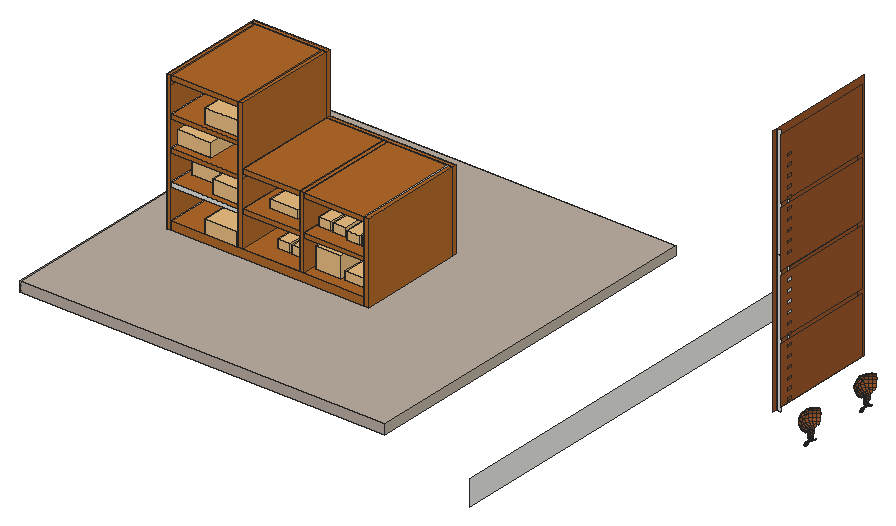
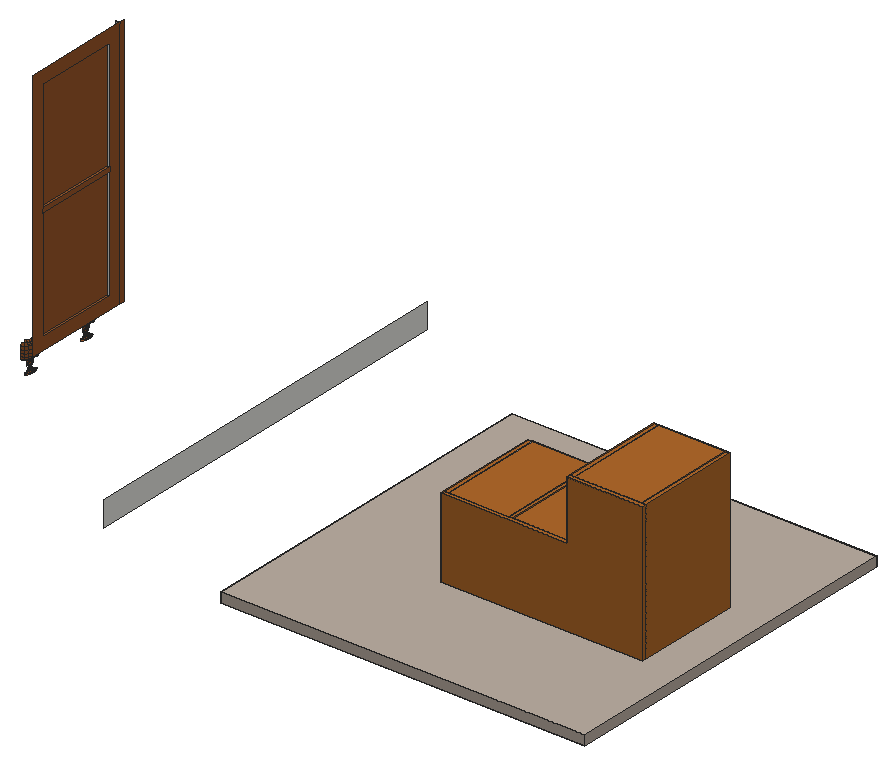
# SketchUp Ruby script. Lengths in inches.
U = 1.inch
M = Sketchup.active_model
def pt(a) = Geom::Point3d.new(a.map { |v| v * U })
def face(e, loops, mat)
  f = e.add_face(loops[0].map { |a| pt(a) })
  loops[1..].each { |l| e.add_face(l.map { |a| pt(a) }).erase! }
  f.material = f.back_material = mat if mat
  f
end
# faces: each face lists its corners as indices into pts; further lists are holes
def faces(e, pts, list, mat = nil) = list.each { |f| face(e, (f[0].is_a?(Array) ? f : [f]).map { |l| l.map { |i| pts[i] } }, mat) }
# xy, xz, yz: faces in a plane at the given z, y or x. An outline is a flat list of corners, or four numbers for a rectangle; further outlines are holes
def ring(l) = l.size == 4 ? [[l[0], l[1]], [l[2], l[1]], [l[2], l[3]], [l[0], l[3]]] : l.each_slice(2).to_a
def flat(e, list, mat, &to3) = list.each { |f| face(e, (f[0].is_a?(Array) ? f : [f]).map { |l| ring(l).map { |u, v| to3.(u, v) } }, mat) }
def xy(e, z, list, mat = nil) = flat(e, list, mat) { |x, y| [x, y, z] }
def xz(e, y, list, mat = nil) = flat(e, list, mat) { |x, z| [x, y, z] }
def yz(e, x, list, mat = nil) = flat(e, list, mat) { |y, z| [x, y, z] }
def lines(e, pts, list) = list.each { |a, b| e.add_line(pt(pts[a]), pt(pts[b])) }
# prism: a flat outline (further loops are holes) pulled along v
def prism(e, loops, v, mat = nil)
  f = face(e, loops, mat); d = Geom::Vector3d.new(v.map { |x| x * U })
  f.pushpull(f.normal.samedirection?(d) ? d.length : -d.length)
end
def box(e, o, s, mat = nil) = prism(e, [[o, [o[0] + s[0], o[1], o[2]], [o[0] + s[0], o[1] + s[1], o[2]], [o[0], o[1] + s[1], o[2]]]], [0, 0, s[2]], mat)
def at(x, y, z, deg = 0) = Geom::Transformation.translation(pt([x, y, z])) * Geom::Transformation.rotation(ORIGIN, Z_AXIS, deg.degrees)
def axes(o, x, y, z) = Geom::Transformation.new([*x, 0, *y, 0, *z, 0, *pt(o).to_a, 1])
def part(name) = M.definitions.add(name)
# library, detail: a bought-in or finely detailed component or shape, given as its bounding box
def library(name, o, s) = part(name).tap { |d| box(d.entities, o, s) }
def detail(e, o, s) = box(e.add_group.entities, o, s)
def put(e, d, t, mat = nil) = e.add_instance(d, t).tap { |i| i.material = mat if mat }
def group(e, t, mat = nil) = e.add_group.tap { |g| g.transformation = t; g.material = mat if mat }.entities
root = M.entities
M.materials.add("[Color A01]").color = [255, 204, 204]
M.materials.add("[Color A07]").color = [153, 0, 0]
M.materials.add("[Color E01]").color = [255, 255, 204]
M.materials.add("[Color G05]").color = [0, 255, 0]
M.materials.add("[Color I01]").color = [204, 204, 255]
M.materials.add("[Color J06]").color = [102, 0, 204]
M.materials.add("[Color K04]").color = [255, 50, 255]
M.materials.add("[Color L11]").color = [153, 0, 76]
M.materials.add("[Color L16]").color = [102, 0, 51]
M.materials.add("[Color M01]").color = [226, 226, 226]
M.materials.add("[Encaustic Tile Circular 02]").color = [187, 174, 162]
M.materials.add("[Wood Bamboo]").color = [177, 105, 43]
M.materials.add("[Wood Cherry Original]").color = [152, 86, 42]
c1 = library("Group\#29",[0,0,0],[10.56,11.41,4.2])
c2 = library("12.1shooters 6",[-12.32,-1,-0.41],[13.09,17.1,6.95])
c3 = library("Group\#37",[0,0,0],[11.84,13.47,5.24])
c4 = library("Group\#20",[0,0,0],[10.15,12.29,4.29])
c5 = library("Group\#27",[0,0,0],[11.1875,13.6,5.13])
c6 = library("Group\#4",[0,0,0],[9.05,3.05,1.93])
c7 = library("Group\#47",[0,0,0],[9.05,6.59,1.93])
c8 = library("Group\#2",[0,0,0],[9.05,3.05,1.93])
c9 = library("Group\#75",[0,0,0],[9.05,3.05,1.93])
c10 = library("ZSHOE",[-0.73,-0.58,0],[16.86,13.33,10.8125])
c11 = library("Group\#12",[0,0,0],[9.05,3.05,1.93])
c12 = library("Group\#3",[0,0,0],[9.05,3.05,1.93])
c13 = library("Group\#44",[0,0,0],[9.05,6.59,1.93])
c14 = library("Group\#73",[0,0,0],[9.05,3.05,1.93])
xy(root,0,[[8.92,47.18,9.92,72.18],[9.92,47.18,9.92,72.18,8.92,72.18,8.92,73.18,56.92,73.18,56.92,72.18,55.92,72.18,55.92,47.18],[55.92,47.18,56.92,72.18]])
xy(root,2,[[25.92,47.18,26.92,72.18],[40.48,47.18,41.48,72.18]])
xy(root,2,[[9.92,47.18,25.92,72.18],[26.92,47.18,40.48,72.18],[41.48,47.18,55.92,72.18]],"[Wood Bamboo]")
xy(root,6,[[159.72,48.4,159.8125,48.51,159.45,48.88,159.33,48.79],[159.33,48.79,159.45,48.88,159.1875,49.33,159.05,49.28],[159.05,49.28,159.1875,49.33,159.06,49.84,158.91,49.82],[158.91,49.82,159.06,49.84,159.06,50.35,158.91,50.375],[159.06,50.35,159.19,50.85,159.06,50.91,158.91,50.375],
  [159.19,50.85,159.46,51.3,159.34,51.4,159.06,50.91],[159.46,51.3,159.82,51.67,159.73,51.79,159.34,51.4],[159.72,65.02,159.8125,65.14,159.45,65.51,159.33,65.42],[159.33,65.42,159.45,65.51,159.1875,65.96,159.05,65.9],[159.05,65.9,159.1875,65.96,159.06,66.46,158.91,66.44],
  [158.91,66.44,159.06,66.46,159.06,66.98,158.91,67],[159.06,66.98,159.19,67.48,159.06,67.54,158.91,67],[159.19,67.48,159.46,67.93,159.34,68.02,159.06,67.54],[159.46,67.93,159.82,68.29,159.73,68.41,159.34,68.02]],"[Wood Cherry Original]")
xy(root,9.25,[[9.92,47.18,25.92,72.18]])
xy(root,9.5,[[41.48,47.18,55.92,72.18]])
xy(root,9.5,[[26.92,47.18,40.48,72.18]],"[Wood Bamboo]")
xy(root,10.25,[[9.92,47.18,25.92,72.18]],"[Wood Bamboo]")
xy(root,10.5,[[26.92,47.18,40.48,72.18],[41.48,47.18,55.92,72.18]],"[Wood Bamboo]")
xy(root,16.08,[[154.9,49.11,155.65,69.11]],"[Wood Cherry Original]")
xy(root,16.5,[[9.92,47.18,25.92,72.18]],"[Wood Bamboo]")
xy(root,17.5,[[9.92,47.18,25.92,72.18]],"[Wood Bamboo]")
xy(root,19,[[26.92,47.18,40.48,72.18],[40.48,47.18,41.48,72.18],[41.48,47.18,55.92,72.18],[55.92,47.18,56.92,72.18],[26.92,72.18,56.92,73.18]],"[Wood Bamboo]")
xy(root,23.75,[[9.92,47.18,25.92,72.18]],"[Wood Bamboo]")
xy(root,24.75,[[9.92,47.18,25.92,72.18]],"[Wood Bamboo]")
xy(root,33,[[8.92,47.18,9.92,72.18],[9.92,47.18,25.92,72.18],[25.92,47.18,26.92,72.18],[8.92,72.18,25.92,73.18],[25.92,72.18,26.92,73.18]],"[Wood Bamboo]")
xy(root,42.58,[[154.9,49.11,155.65,69.11]],"[Wood Cherry Original]")
xy(root,43.58,[[154.9,49.11,155.65,69.11]],"[Wood Cherry Original]")
xy(root,70.08,[[154.9,49.11,155.65,69.11]])
xz(root,46.11,[[154.9,13.08,155.9,46.26],[154.9,46.26,155.9,73.08]])
xz(root,47.18,[[9.92,9.25,25.92,10.25]])
xz(root,47.18,[[8.92,0,9.92,33],[9.92,0,55.92,2],[55.92,0,56.92,19],[25.92,2,26.92,33],[40.48,2,41.48,19],
  [26.92,9.5,40.48,10.5],[41.48,9.5,55.92,10.5],[9.92,16.5,25.92,17.5],[26.92,18,40.48,19],[41.48,18,55.92,19],
  [9.92,23.75,25.92,24.75],[9.92,32,25.92,33]],"[Wood Bamboo]")
xz(root,49.11,[[154.9,16.08,155.65,42.58],[154.9,43.58,155.65,70.08]])
xz(root,69.11,[[154.9,16.08,155.65,42.58],[154.9,43.58,155.65,70.08]],"[Wood Cherry Original]")
xz(root,72.18,[[8.92,0,9.92,33],[55.92,0,56.92,19],[25.92,2,26.92,33],[40.48,2,41.48,2,41.48,17,26.92,17,26.92,9.5,40.48,9.5],[9.92,9.25,25.92,31],
  [41.48,9.5,55.92,17],[26.92,17,40.48,19],[40.48,17,41.48,19],[41.48,17,55.92,19],[9.92,17.5,25.92,23.75],
  [9.92,31,25.92,33]])
xz(root,72.18,[[9.92,2,25.92,9.25],[26.92,2,40.48,9.5],[41.48,2,55.92,9.5],[9.92,10.25,25.92,16.5],[26.92,10.5,40.48,17],
  [41.48,10.5,55.92,17],[9.92,24.75,25.92,31]],"[Wood Bamboo]")
xz(root,73.18,[[8.92,0,8.92,33,26.92,33,26.92,19,56.92,19,56.92,0]],"[Wood Bamboo]")
yz(root,8.92,[[47.18,0,72.18,33],[72.18,0,73.18,33]],"[Wood Bamboo]")
yz(root,9.92,[[47.18,0,72.18,2],[47.18,9.25,72.18,10.25],[47.18,16.5,72.18,17.5],[47.18,23.75,72.18,24.75]])
yz(root,9.92,[[47.18,2,72.18,9.25],[47.18,10.25,72.18,16.5],[47.18,17.5,72.18,23.75],[47.18,24.75,72.18,31],[47.18,31,72.18,33]],"[Wood Bamboo]")
yz(root,25.92,[[47.18,2,72.18,9.25],[47.18,9.25,72.18,10.25],[47.18,16.5,72.18,17.5],[47.18,23.75,72.18,24.75]])
yz(root,25.92,[[47.18,10.25,72.18,16.5],[47.18,17.5,72.18,23.75],[47.18,24.75,72.18,31],[47.18,31,72.18,33]],"[Wood Bamboo]")
yz(root,26.92,[[47.18,9.5,72.18,10.5]])
yz(root,26.92,[[47.18,2,72.18,9.5],[47.18,10.5,72.18,17],[47.18,17,72.18,19],[47.18,19,72.18,33],[72.18,19,73.18,33]],"[Wood Bamboo]")
yz(root,40.48,[[47.18,2,72.18,9.5],[47.18,10.5,72.18,19]],"[Wood Bamboo]")
yz(root,41.48,[[47.18,9.5,72.18,10.5]])
yz(root,41.48,[[47.18,2,72.18,9.5],[47.18,10.5,72.18,19]],"[Wood Bamboo]")
yz(root,55.92,[[47.18,0,72.18,2],[47.18,9.5,72.18,10.5],[47.18,17,72.18,19]])
yz(root,55.92,[[47.18,2,72.18,9.5],[47.18,10.5,72.18,17]],"[Wood Bamboo]")
yz(root,56.92,[[47.18,0,72.18,19],[72.18,0,73.18,19]],"[Wood Bamboo]")
yz(root,118.75,[[0,0,96.25,6]])
yz(root,154.9,[[45.11,13.08,46.11,73.08],[[46.11,13.08,72.11,73.08],[49.11,16.08,69.11,70.08]],[49.11,42.58,69.11,43.58]],"[Wood Cherry Original]")
yz(root,155.65,[[49.11,16.08,69.11,42.58],[49.11,43.58,69.11,70.08]],"[Wood Cherry Original]")
yz(root,155.9,[[46.11,14.08,70.11,27.58],[46.11,28.58,70.11,42.08],[46.11,43.08,70.11,56.58],[46.11,57.58,70.11,72.08]],"[Wood Cherry Original]")
yz(root,158.4,[[45.11,35.1,46.11,35.6],[45.11,37.43,46.11,37.93],[45.11,39.75,46.11,40.25],[45.11,42.08,46.11,42.58]])
yz(root,158.4,[[45.11,16.73,46.11,17.26],[45.11,18.83,46.11,19.33],[45.11,21.15,46.11,21.65],[45.11,23.48,46.11,23.98],[45.11,25.8,46.11,26.3],
  [45.11,28.125,46.11,28.625],[45.11,30.45,46.11,30.95],[45.11,32.78,46.11,33.28],[45.11,47.97,46.11,48.47],[45.11,50.29,46.11,50.79],
  [45.11,52.62,46.11,53.12],[45.11,54.94,46.11,55.44],[45.11,57.27,46.11,57.77],[45.11,59.59,46.11,60.09],[45.11,61.92,46.11,62.42],
  [45.11,64.24,46.11,64.74],[45.11,66.57,46.11,67.07],[45.11,68.89,46.11,69.39]],"[Wood Cherry Original]")
yz(root,159.53,[[49.9,8.1,50.29,8.4],[66.52,8.1,66.52,8.4,66.92,8.4,66.91,8.1]],"[Wood Cherry Original]")
yz(root,159.84,[[49.93,6.79,50.25,6.94],[66.56,6.79,66.875,6.94]],"[Wood Cherry Original]")
p = [[159.57,48.97,6.03],[159.45,48.88,6],[159.8125,48.51,6],[159.9,48.63,6.03],[159.68,49.06,6.08],[159.99,48.75,6.08],
  [159.33,49.39,6.03],[159.1875,49.33,6],[159.46,49.44,6.08],[159.2,49.85,6.03],[159.06,49.84,6],[159.34,49.87,6.08],
  [159.21,50.33,6.03],[159.06,50.35,6],[159.35,50.32,6.08],[159.33,50.8,6.03],[159.19,50.85,6],[159.46,50.74,6.08],
  [159.6875,51.125,6.08],[159.57,51.21,6.03],[159.46,51.3,6],[160,51.4375,6.08],[159.91,51.55,6.03],[159.82,51.67,6],
  [159.57,65.6,6.03],[159.45,65.51,6],[159.8125,65.14,6],[159.9,65.26,6.03],[159.68,65.68,6.08],[159.99,65.37,6.08],
  [159.33,66.02,6.03],[159.1875,65.96,6],[159.46,66.07,6.08],[159.2,66.48,6.03],[159.06,66.46,6],[159.34,66.5,6.08],
  [159.21,66.96,6.03],[159.06,66.98,6],[159.35,66.94,6.08],[159.46,67.37,6.08],[159.33,67.42,6.03],[159.19,67.48,6],
  [159.57,67.84,6.03],[159.46,67.93,6],[159.6875,67.75,6.08],[159.91,68.18,6.03],[159.82,68.29,6],[160,68.0625,6.08],
  [159.78,49.14,6.16],[160.07,48.85,6.16],[159.58,49.49,6.16],[159.47,49.89,6.16],[159.48,50.3,6.16],[159.58,50.69,6.16],
  [159.79,51.05,6.16],[159.78,65.76,6.16],[160.07,65.47,6.16],[159.58,66.12,6.16],[159.47,66.51,6.16],[159.48,66.92,6.16],
  [159.58,67.32,6.16],[159.79,67.67,6.16],[159.6875,49.54,6.25],[159.875,49.21,6.25],[159.59,49.9,6.25],[159.59,50.28,6.25],
  [159.69,50.65,6.25],[159.88,50.97,6.25],[159.6875,66.16,6.25],[159.875,65.83,6.25],[159.59,66.53,6.25],[159.59,66.91,6.25],
  [159.69,67.27,6.25],[159.88,67.6,6.25],[159.78,49.57,6.37],[159.95,49.27,6.37],[159.68,49.92,6.37],[159.6875,50.27,6.37],
  [159.78,50.61,6.37],[159.96,50.92,6.37],[159.78,66.2,6.37],[159.95,65.89,6.37],[159.68,66.54,6.37],[159.6875,66.89,6.37],
  [159.78,67.24,6.37],[159.96,67.54,6.37],[159.76,49.93,6.5],[159.84,49.6,6.5],[159.76,50.26,6.5],[159.85,50.58,6.5],
  [159.76,66.55,6.5],[159.84,66.23,6.5],[159.76,66.88,6.5],[159.85,67.21,6.5],[159.81,49.93,6.64],[159.89,49.62,6.64],
  [159.8125,50.25,6.64],[159.9,50.5625,6.64],[159.81,66.56,6.64],[159.89,66.25,6.64],[159.8125,66.88,6.64],[159.9,67.1875,6.64],
  [159.84,49.93,6.79],[159.92,49.63,6.79],[159.84,50.25,6.79],[159.92,50.55,6.79],[159.84,66.56,6.79],[159.92,66.26,6.79],
  [159.84,66.875,6.79],[159.92,67.18,6.79],[159.84,49.93,6.94],[159.92,49.63,6.94],[159.92,50.55,6.94],[159.84,50.25,6.94],
  [159.84,66.56,6.94],[159.92,66.26,6.94],[159.92,67.18,6.94],[159.84,66.875,6.94],[159.81,49.93,7.09],[159.89,49.62,7.09],
  [159.8125,50.25,7.09],[159.89,50.5625,7.09],[159.81,66.56,7.09],[159.89,66.25,7.09],[159.8125,66.88,7.09],[159.89,67.1875,7.09],
  [159.76,49.92,7.23],[159.84,49.6,7.23],[159.76,50.26,7.23],[159.85,50.58,7.23],[159.76,66.55,7.23],[159.84,66.23,7.23],
  [159.76,66.88,7.23],[159.85,67.21,7.23],[159.74,49.56,7.51],[160.01,49.3125,7.23],[159.92,49.24,7.51],[159.65,49.91,7.51],
  [159.65,50.27,7.51],[159.74,50.625,7.51],[159.74,66.18,7.51],[160.01,65.9375,7.23],[159.92,65.87,7.51],[159.65,66.54,7.51],
  [159.65,66.9,7.51],[159.74,67.25,7.51],[159.67,49.53,7.8],[159.86,49.2,7.8],[159.57,49.9,7.8],[159.57,50.28,7.8],
  [159.67,50.65,7.8],[159.87,50.98,7.8],[159.93,50.9375,7.51],[159.67,66.16,7.8],[159.86,65.82,7.8],[159.57,66.53,7.8],
  [159.57,66.91,7.8],[159.67,67.28,7.8],[159.87,67.61,7.8],[159.93,67.5625,7.51],[159.63,49.52,8.1],[159.83,49.17,8.1],
  [159.53,49.9,8.1],[159.53,50.29,8.1],[159.64,50.67,8.1],[159.84,51.01,8.1],[159.63,66.14,8.1],[159.83,65.8,8.1],
  [159.53,66.52,8.1],[159.53,66.91,8.1],[159.64,67.29,8.1],[159.84,67.63,8.1],[159.63,49.51,8.4],[159.83,49.17,8.4],
  [159.53,49.9,8.4],[159.64,50.67,8.4],[159.53,50.29,8.4],[159.83,51.01,8.4],[159.63,66.14,8.4],[159.83,65.8,8.4],
  [159.53,66.52,8.4],[159.64,67.3,8.4],[159.53,66.92,8.4],[159.83,67.64,8.4],[159.66,49.53,8.7],[159.85,49.19,8.7],
  [159.5625,49.9,8.7],[159.57,50.29,8.7],[159.67,50.66,8.7],[159.86,50.99,8.7],[159.66,66.15,8.7],[159.85,65.82,8.7],
  [159.5625,66.53,8.7],[159.57,66.91,8.7],[159.67,67.28,8.7],[159.86,67.62,8.7],[159.73,49.55,8.99],[159.91,49.24,8.99],
  [159.63,49.91,8.99],[159.64,50.28,8.99],[159.73,50.63,8.99],[159.92,50.95,8.99],[159.73,66.18,8.99],[159.91,65.86,8.99],
  [159.63,66.53,8.99],[159.64,66.9,8.99],[159.73,67.26,8.99],[159.92,67.57,8.99],[159.35,48.81,9.21],[160.17,48.98,8.99],
  [159.74,48.42,9.21],[159.08,49.29,9.21],[158.9375,49.82,9.21],[158.9375,50.37,9.21],[159.08,50.9,9.21],[159.36,51.375,9.21],
  [159.75,51.76,9.21],[160.18,51.21,8.99],[159.35,65.44,9.21],[160.17,65.6,8.99],[159.74,65.04,9.21],[159.08,65.91,9.21],
  [158.9375,66.45,9.21],[158.9375,67,9.21],[159.08,67.53,9.21],[159.36,68,9.21],[159.75,68.39,9.21],[160.18,67.83,8.99],
  [159.38,47.96,9.66],[160.21,48.14,9.21],[159.99,47.61,9.66],[158.89,48.46,9.66],[158.54,49.07,9.66],[158.36,49.75,9.66],
  [158.37,50.45,9.66],[158.55,51.125,9.66],[158.9,51.73,9.66],[159.4,52.23,9.66],[160.01,52.57,9.66],[160.23,52.04,9.21],
  [159.38,64.59,9.66],[160.21,64.77,9.21],[159.99,64.23,9.66],[158.89,65.08,9.66],[158.54,65.69,9.66],[158.36,66.37,9.66],
  [158.37,67.07,9.66],[158.55,67.75,9.66],[158.9,68.36,9.66],[159.4,68.85,9.66],[160.01,69.2,9.66],[160.23,68.66,9.21],
  [159.15,47.66,10.28],[159.84,47.26,10.28],[158.59,48.23,10.28],[158.19,48.92,10.28],[157.99,49.7,10.28],[157.99,50.5,10.28],
  [158.2,51.27,10.28],[158.6,51.96,10.28],[159.17,52.53,10.28],[159.87,52.93,10.28],[159.15,64.29,10.28],[159.84,63.88,10.28],
  [158.59,64.85,10.28],[158.19,65.55,10.28],[157.99,66.32,10.28],[157.99,67.125,10.28],[158.2,67.9,10.28],[158.6,68.59,10.28],
  [159.17,69.15,10.28],[159.87,69.55,10.28],[159.07,47.56,11],[159.79,47.14,11],[158.48,48.15,11],[158.07,48.875,11],
  [157.85,49.68,11],[157.86,50.52,11],[158.08,51.32,11],[158.5,52.04,11],[159.09,52.63,11],[159.81,53.05,11],
  [159.07,64.18,11],[159.79,63.76,11],[158.48,64.77,11],[158.07,65.5,11],[157.85,66.31,11],[157.86,67.14,11],
  [158.08,67.95,11],[158.5,68.67,11],[159.09,69.26,11],[159.81,69.67,11],[159.15,47.66,11.72],[159.84,47.26,11.72],
  [158.59,48.23,11.72],[158.19,48.92,11.72],[157.99,49.7,11.72],[157.99,50.5,11.72],[158.2,51.27,11.72],[158.6,51.96,11.72],
  [159.17,52.53,11.72],[159.87,52.93,11.72],[159.15,64.29,11.72],[159.84,63.88,11.72],[158.59,64.85,11.72],[158.19,65.55,11.72],
  [157.99,66.32,11.72],[157.99,67.125,11.72],[158.2,67.9,11.72],[158.6,68.59,11.72],[159.17,69.15,11.72],[159.87,69.55,11.72],
  [159.38,47.96,12.34],[159.99,47.61,12.34],[158.89,48.46,12.34],[158.54,49.07,12.34],[158.36,49.75,12.34],[158.37,50.45,12.34],
  [158.55,51.125,12.34],[158.9,51.73,12.34],[159.4,52.23,12.34],[160.01,52.57,12.34],[159.38,64.59,12.34],[159.99,64.23,12.34],
  [158.89,65.08,12.34],[158.54,65.69,12.34],[158.36,66.37,12.34],[158.37,67.07,12.34],[158.55,67.75,12.34],[158.9,68.36,12.34],
  [159.4,68.85,12.34],[160.01,69.2,12.34],[159.74,48.42,12.79],[160.21,48.14,12.79],[159.35,48.81,12.79],[159.08,49.29,12.79],
  [158.9375,49.82,12.79],[158.9375,50.37,12.79],[159.08,50.9,12.79],[159.36,51.375,12.79],[159.75,51.76,12.79],[160.23,52.04,12.79],
  [159.74,65.04,12.79],[160.21,64.77,12.79],[159.35,65.44,12.79],[159.08,65.91,12.79],[158.9375,66.45,12.79],[158.9375,67,12.79],
  [159.08,67.53,12.79],[159.36,68,12.79],[159.75,68.39,12.79],[160.23,68.66,12.79],[159.91,49.24,13.01],[160.17,48.98,13.01],
  [159.73,49.55,13.01],[159.63,49.91,13.01],[159.64,50.28,13.01],[159.73,50.63,13.01],[159.92,50.95,13.01],[160.18,51.21,13.01],
  [159.91,65.86,13.01],[160.17,65.6,13.01],[159.73,66.18,13.01],[159.63,66.53,13.01],[159.64,66.9,13.01],[159.73,67.26,13.01],
  [159.92,67.57,13.01],[160.18,67.83,13.01]]
faces(root,p,[[0,1,2,3],[4,0,3,5],[6,7,1,0],[8,6,0,4],[9,10,7,6],[11,9,6,8],[12,13,10,9],[14,12,9,11],
  [15,16,13,12],[17,15,12,14],[18,19,15,17],[19,20,16,15],[21,22,19,18],[22,23,20,19],[24,25,26,27],[28,24,27,29],
  [30,31,25,24],[32,30,24,28],[33,34,31,30],[35,33,30,32],[36,37,34,33],[38,36,33,35],[39,40,36,38],[40,41,37,36],
  [42,43,41,40],[44,42,40,39],[45,46,43,42],[47,45,42,44],[48,4,5,49],[50,8,4,48],[51,11,8,50],[52,14,11,51],
  [53,17,14,52],[54,18,17,53],[55,28,29,56],[57,32,28,55],[58,35,32,57],[59,38,35,58],[60,39,38,59],[61,44,39,60],
  [62,50,48,63],[64,51,50,62],[65,52,51,64],[66,53,52,65],[67,54,53,66],[68,57,55,69],[70,58,57,68],[71,59,58,70],
  [72,60,59,71],[73,61,60,72],[74,62,63,75],[76,64,62,74],[77,65,64,76],[78,66,65,77],[79,67,66,78],[80,68,69,81],
  [82,70,68,80],[83,71,70,82],[84,72,71,83],[85,73,72,84],[86,76,74,87],[88,77,76,86],[89,78,77,88],[90,82,80,91],
  [92,83,82,90],[93,84,83,92],[94,86,87,95],[96,88,86,94],[97,89,88,96],[98,90,91,99],[100,92,90,98],[101,93,92,100],
  [102,94,95,103],[104,96,94,102],[105,97,96,104],[106,98,99,107],[108,100,98,106],[109,101,100,108],[110,102,103,111],[112,105,104,113],
  [114,106,107,115],[116,109,108,117],[118,110,111,119],[120,113,110,118],[121,112,113,120],[122,114,115,123],[124,117,114,122],[125,116,117,124],
  [126,118,119,127],[128,120,118,126],[129,121,120,128],[130,122,123,131],[132,124,122,130],[133,125,124,132],[134,127,135,136],[137,126,127,134],
  [138,128,126,137],[139,129,128,138],[140,131,141,142],[143,130,131,140],[144,132,130,143],[145,133,132,144],[146,134,136,147],[148,137,134,146],
  [149,138,137,148],[150,139,138,149],[151,152,139,150],[153,140,142,154],[155,143,140,153],[156,144,143,155],[157,145,144,156],[158,159,145,157],
  [160,146,147,161],[162,148,146,160],[163,149,148,162],[164,150,149,163],[165,151,150,164],[166,153,154,167],[168,155,153,166],[169,156,155,168],
  [170,157,156,169],[171,158,157,170],[172,160,161,173],[174,162,160,172],[175,164,163,176],[177,165,164,175],[178,166,167,179],[180,168,166,178],
  [181,170,169,182],[183,171,170,181],[184,172,173,185],[186,174,172,184],[187,176,174,186],[188,175,176,187],[189,177,175,188],[190,178,179,191],
  [192,180,178,190],[193,182,180,192],[194,181,182,193],[195,183,181,194],[196,184,185,197],[198,186,184,196],[199,187,186,198],[200,188,187,199],
  [201,189,188,200],[202,190,191,203],[204,192,190,202],[205,193,192,204],[206,194,193,205],[207,195,194,206],[208,197,209,210],[211,196,197,208],
  [212,198,196,211],[213,199,198,212],[214,200,199,213],[215,201,200,214],[216,217,201,215],[218,203,219,220],[221,202,203,218],[222,204,202,221],
  [223,205,204,222],[224,206,205,223],[225,207,206,224],[226,227,207,225],[228,210,229,230],[231,208,210,228],[232,211,208,231],[233,212,211,232],
  [234,213,212,233],[235,214,213,234],[236,215,214,235],[237,216,215,236],[238,239,216,237],[240,220,241,242],[243,218,220,240],[244,221,218,243],
  [245,222,221,244],[246,223,222,245],[247,224,223,246],[248,225,224,247],[249,226,225,248],[250,251,226,249],[252,228,230,253],[254,231,228,252],
  [255,232,231,254],[256,233,232,255],[257,234,233,256],[258,235,234,257],[259,236,235,258],[260,237,236,259],[261,238,237,260],[262,240,242,263],
  [264,243,240,262],[265,244,243,264],[266,245,244,265],[267,246,245,266],[268,247,246,267],[269,248,247,268],[270,249,248,269],[271,250,249,270],
  [272,252,253,273],[274,254,252,272],[275,255,254,274],[276,256,255,275],[277,257,256,276],[278,258,257,277],[279,259,258,278],[280,260,259,279],
  [281,261,260,280],[282,262,263,283],[284,264,262,282],[285,265,264,284],[286,266,265,285],[287,267,266,286],[288,268,267,287],[289,269,268,288],
  [290,270,269,289],[291,271,270,290],[292,272,273,293],[294,274,272,292],[295,275,274,294],[296,276,275,295],[297,277,276,296],[298,278,277,297],
  [299,279,278,298],[300,280,279,299],[301,281,280,300],[302,282,283,303],[304,284,282,302],[305,285,284,304],[306,286,285,305],[307,287,286,306],
  [308,288,287,307],[309,289,288,308],[310,290,289,309],[311,291,290,310],[312,292,293,313],[314,294,292,312],[315,295,294,314],[316,296,295,315],
  [317,297,296,316],[318,298,297,317],[319,299,298,318],[320,300,299,319],[321,301,300,320],[322,302,303,323],[324,304,302,322],[325,305,304,324],
  [326,306,305,325],[327,307,306,326],[328,308,307,327],[329,309,308,328],[330,310,309,329],[331,311,310,330],[332,312,313,333],[334,314,312,332],
  [335,315,314,334],[336,316,315,335],[337,317,316,336],[338,318,317,337],[339,319,318,338],[340,320,319,339],[341,321,320,340],[342,322,323,343],
  [344,324,322,342],[345,325,324,344],[346,326,325,345],[347,327,326,346],[348,328,327,347],[349,329,328,348],[350,330,329,349],[351,331,330,350],
  [352,334,332,353],[354,335,334,352],[355,336,335,354],[356,337,336,355],[357,338,337,356],[358,339,338,357],[359,340,339,358],[360,344,342,361],
  [362,345,344,360],[363,346,345,362],[364,347,346,363],[365,348,347,364],[366,349,348,365],[367,350,349,366]],"[Wood Cherry Original]")
put(root,c1,axes([9.9,49.06,17.5],[0.7668,0,0],[0,0.7668,0],[0,0,0.7668]),"[Color J06]")
put(root,c2,axes([17.38,52.41,10.25],[0.51,0,0],[0,0.51,0],[0,0,0.51]),"[Color L11]")
put(root,c3,axes([17.21,48.2,24.75],[0.67,0,0],[0,0.67,0],[0,0,0.67]),"[Color A07]")
put(root,c4,axes([17.92,47.18,2],[0.7455,0,0],[0,0.7455,0],[0,0,0.7455]),"[Color A07]")
put(root,c5,axes([18.82,48.43,10.25],[0.62,0,0],[0,0.62,0],[0,0,0.62]),"[Color L16]")
put(root,c6,axes([31.89,51.375,2],[0,1,0],[1,0,0],[0,0,1]),"[Color A01]")
put(root,c7,axes([30.77,50.57,10.5],[0,1,0],[1,0,0],[0,0,1]),"[Color E01]")
put(root,c8,at(38.48,51.375,2,90),"[Color A01]")
g1 = group(root,at(0,14.77,-2.4375),"[Encaustic Tile Circular 02]")
box(g1,[0,0,0],[86.6875,86.6875,2.3125])
put(root,c9,axes([42.03,50.92,10.5],[0,1,0],[1,0,0],[0,0,1]),"[Color M01]")
put(root,c10,axes([42.59,56.92,2],[0,-0.44906,0],[0.44906,0,0],[0,0,0.44906]),"[Color I01]")
put(root,c11,at(48.61,50.92,10.5,90),"[Color M01]")
put(root,c12,axes([49.33,50.21,10.5],[0,1,0],[1,0,0],[0,0,1]),"[Color G05]")
put(root,c13,at(55.92,49.78,2,90),"[Color K04]")
put(root,c14,at(55.92,50.21,10.5,90),"[Color G05]")
